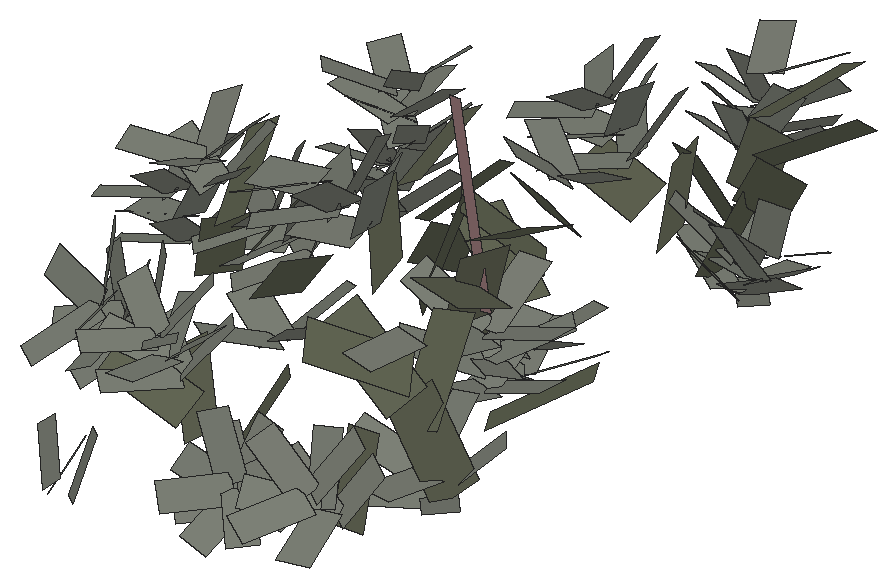
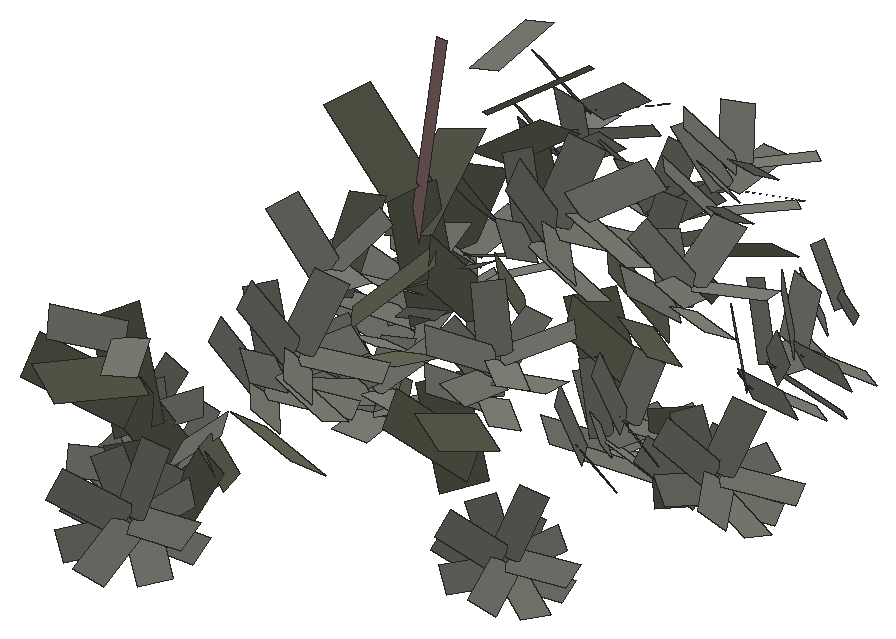
# SketchUp Ruby script. Lengths in inches.
U = 1.inch
M = Sketchup.active_model
def pt(a) = Geom::Point3d.new(a.map { |v| v * U })
def face(e, loops, mat)
  f = e.add_face(loops[0].map { |a| pt(a) })
  loops[1..].each { |l| e.add_face(l.map { |a| pt(a) }).erase! }
  f.material = f.back_material = mat if mat
  f
end
# faces: each face lists its corners as indices into pts; further lists are holes
def faces(e, pts, list, mat = nil) = list.each { |f| face(e, (f[0].is_a?(Array) ? f : [f]).map { |l| l.map { |i| pts[i] } }, mat) }
# xy, xz, yz: faces in a plane at the given z, y or x. An outline is a flat list of corners, or four numbers for a rectangle; further outlines are holes
def ring(l) = l.size == 4 ? [[l[0], l[1]], [l[2], l[1]], [l[2], l[3]], [l[0], l[3]]] : l.each_slice(2).to_a
def flat(e, list, mat, &to3) = list.each { |f| face(e, (f[0].is_a?(Array) ? f : [f]).map { |l| ring(l).map { |u, v| to3.(u, v) } }, mat) }
def xy(e, z, list, mat = nil) = flat(e, list, mat) { |x, y| [x, y, z] }
def xz(e, y, list, mat = nil) = flat(e, list, mat) { |x, z| [x, y, z] }
def yz(e, x, list, mat = nil) = flat(e, list, mat) { |y, z| [x, y, z] }
def lines(e, pts, list) = list.each { |a, b| e.add_line(pt(pts[a]), pt(pts[b])) }
# prism: a flat outline (further loops are holes) pulled along v
def prism(e, loops, v, mat = nil)
  f = face(e, loops, mat); d = Geom::Vector3d.new(v.map { |x| x * U })
  f.pushpull(f.normal.samedirection?(d) ? d.length : -d.length)
end
def box(e, o, s, mat = nil) = prism(e, [[o, [o[0] + s[0], o[1], o[2]], [o[0] + s[0], o[1] + s[1], o[2]], [o[0], o[1] + s[1], o[2]]]], [0, 0, s[2]], mat)
def at(x, y, z, deg = 0) = Geom::Transformation.translation(pt([x, y, z])) * Geom::Transformation.rotation(ORIGIN, Z_AXIS, deg.degrees)
def axes(o, x, y, z) = Geom::Transformation.new([*x, 0, *y, 0, *z, 0, *pt(o).to_a, 1])
def part(name) = M.definitions.add(name)
# library, detail: a bought-in or finely detailed component or shape, given as its bounding box
def library(name, o, s) = part(name).tap { |d| box(d.entities, o, s) }
def detail(e, o, s) = box(e.add_group.entities, o, s)
def put(e, d, t, mat = nil) = e.add_instance(d, t).tap { |i| i.material = mat if mat }
def group(e, t, mat = nil) = e.add_group.tap { |g| g.transformation = t; g.material = mat if mat }.entities
root = M.entities
M.materials.add("tak1dsfasd0f156w").color = [150, 118, 119]
M.materials.add("viburnumblaasdfas0df1w06d").color = [98, 102, 84]
M.materials.add("viburnumbladsadfasdfad0w122").color = [125, 129, 119]
c1 = part("Component\#315")
p = [[0.25,0,0],[2.05,0.01,0.35],[1.81,4.2,1.66],[0,4.19,1.3125]]
faces(c1.entities,p,[[0,1,2,3]],"viburnumbladsadfasdfad0w122")
c2 = part("viburnumblad2")
put(c2.entities,c1,axes([-19.23,-4.49,-32.18],[83.35428,0,0],[0,79.38502,0],[0,0,83.35428]))
c3 = part("Component\#314")
p = [[0.14,0,0],[2.58,0.05,0.25],[2.44,5.11,2.64],[0,5.05,2.39]]
faces(c3.entities,p,[[0,1,2,3]],"viburnumblaasdfas0df1w06d")
c4 = part("viburnumblad1\#2")
put(c4.entities,c3,axes([-37.25,6.23,19.31],[75.98784,0,0],[0,65.50676,0],[0,0,75.98784]))
c5 = part("Component\#337")
p = [[0.6,0,12.07],[1.51,1.22,0.03],[0.91,1.23,0],[0,0,12.04]]
faces(c5.entities,p,[[0,1,2,3]],"tak1dsfasd0f156w")
put(root,c2,axes([1233.48,261.68,34.33],[-0.00995,0.00489,0.00397],[-0.00628,-0.00876,-0.0047],[0.00102,-0.00608,0.00892]))
put(root,c2,axes([1233.86,263.27,33.78],[-0.01153,-0.00217,-0.00126],[0.00257,-0.00998,-0.00587],[-0.00007,-0.00594,0.00905]))
put(root,c2,axes([1227.22,263.09,31.97],[-0.00593,0.00534,0.00783],[-0.0086,-0.00691,-0.00181],[0.00397,-0.00698,0.00778]))
put(root,c2,axes([1232.86,262.36,33.13],[-0.00254,0.00908,0.00688],[-0.01141,-0.00302,-0.00024],[0.00165,-0.00679,0.00837]))
put(root,c2,axes([1227.72,264.1,32.82],[-0.00902,-0.00601,-0.00274],[0.00624,-0.00625,-0.00686],[0.00215,-0.00706,0.0084]))
put(root,c2,axes([1231.99,261.6,34.32],[0.00636,0.00796,0.00575],[-0.00984,0.00398,0.00495],[0.00146,-0.00765,0.00773]))
put(root,c2,axes([1215.61,263.46,29.77],[0.00345,-0.00905,-0.004],[0.00788,-0.00012,0.00668],[-0.00594,-0.00519,0.00581]))
put(root,c2,axes([1227.25,264.68,31.45],[-0.01058,-0.00047,0.0036],[-0.00191,-0.00936,-0.00683],[0.00314,-0.00674,0.00835]))
put(root,c2,axes([1231.93,262.78,35.2],[0.00995,-0.00489,-0.00397],[0.00634,0.00703,0.00672],[-0.00053,-0.00802,0.00751]))
put(root,c2,axes([1214.98,262.74,28.87],[0.00855,0.00051,0.00592],[-0.00403,0.00835,0.00477],[-0.00448,-0.00623,0.00604]))
put(root,c2,axes([1226.24,263.93,31.04],[0.00218,0.00802,0.00747],[-0.00931,-0.0013,0.00412],[0.00416,-0.00766,0.007]))
put(root,c2,axes([1225.95,263.21,32.57],[0.00902,0.00601,0.00274],[-0.00554,0.00435,0.00868],[0.0036,-0.00837,0.00649]))
put(root,c2,axes([1226.29,265,30.18],[-0.0062,0.00558,0.00817],[-0.00774,-0.00622,-0.00163],[0.00397,-0.00698,0.00778]))
put(root,c2,axes([1215.79,263.78,28.39],[0.00848,-0.00604,0.00136],[0.00312,0.00638,0.00815],[-0.00533,-0.00595,0.00568]))
put(root,c2,axes([1231.8,263,33.61],[0.01153,0.00217,0.00126],[-0.00261,0.00855,0.00823],[0.00055,-0.00816,0.00738]))
put(root,c2,axes([1232.29,263.4375,32.28],[0.00611,0.00764,0.00552],[-0.01063,0.0043,0.00535],[0.00146,-0.00765,0.00773]))
put(root,c2,axes([1226.45,264.22,33.43],[0.00593,-0.00534,-0.00783],[0.00931,0.00502,0.00364],[0.00177,-0.00845,0.00711]))
put(root,c2,axes([1226.68,265.32,32.37],[-0.00218,-0.00802,-0.00747],[0.01085,-0.00048,-0.00266],[0.00158,-0.00777,0.00788]))
put(root,c2,axes([1220.38,265.37,37.75],[-0.00773,0.00806,0.00054],[-0.00787,-0.00734,-0.00302],[-0.00183,-0.00247,0.01075]))
put(root,c2,axes([1221.09,266.52,36.78],[-0.01083,0.00076,-0.00267],[-0.00024,-0.01097,-0.00215],[-0.00276,-0.00202,0.01064]))
put(root,c2,axes([1220.6,266.68,38.24],[-0.00759,-0.00699,-0.00431],[0.00733,-0.00841,0.00072],[-0.00369,-0.00233,0.01029]))
put(root,c2,axes([1232.09,264.59,33.1875],[0.01038,-0.0051,-0.00415],[0.00571,0.00633,0.00604],[-0.00053,-0.00802,0.00751]))
put(root,c2,axes([1225.42,264.67,32.17],[0.01058,0.00047,-0.0036],[0.00255,0.00709,0.00842],[0.00261,-0.00869,0.00653]))
put(root,c2,axes([1221.08,266.54,35.28],[-0.00742,0.00774,0.00052],[-0.0085,-0.00793,-0.00326],[-0.00183,-0.00247,0.01075]))
put(root,c2,axes([1225.21,264.99,30.72],[0.0079,0.00633,0.00186],[-0.00554,0.00435,0.00868],[0.00455,-0.00767,0.00675]))
put(root,c2,axes([1220.16,265.82,36.28],[-0.0001,0.01064,0.00343],[-0.01164,0.00037,-0.00146],[-0.00143,-0.00341,0.01055]))
put(root,c4,axes([1231.6875,266,30.82],[0.01273,-0.00184,0.00122],[0.00029,0.0105,0.01027],[-0.0024,-0.00896,0.00784]))
put(root,c2,axes([1220.25,267.68,36.92],[0.0001,-0.01064,-0.00343],[0.01052,-0.00118,0.00394],[-0.00407,-0.00322,0.0099]))
put(root,c2,axes([1219.03,265.7,37.5],[0.00759,0.00699,0.00431],[-0.00801,0.0076,0.00179],[-0.00181,-0.0043,0.01016]))
put(root,c2,axes([1219.25,267,37.98],[0.00773,-0.00806,-0.00054],[0.0072,0.00653,0.00553],[-0.00368,-0.00417,0.0097]))
put(root,c4,axes([1220.77,267.16,32.375],[0.0023,0.0101,0.00657],[-0.0138,0.00343,-0.00044],[-0.0019,-0.0063,0.01035]))
put(root,c2,axes([1219.1875,266.71,36.29],[0.01083,-0.00076,0.00267],[-0.0004,0.00932,0.00428],[-0.00274,-0.00461,0.00981]))
put(root,c2,axes([1233.8,270.26,40.56],[-0.01204,0.00026,0.00058],[-0.00039,-0.0134,-0.00212],[0.00055,-0.00198,0.01239]))
put(root,c2,axes([1219.7,266.74,35.01],[0.00793,0.00729,0.0045],[-0.00721,0.00684,0.00161],[-0.00181,-0.0043,0.01016]))
put(root,c2,axes([1219.8125,267.84,35.5],[0.00743,-0.00696,-0.00145],[0.0072,0.00653,0.00553],[-0.00282,-0.00502,0.00959]))
put(root,c4,axes([1233.05,270.12,37.29],[-0.00623,0.01061,0.0062],[-0.01365,-0.00831,0.0005],[0.00356,-0.0051,0.0123]))
put(root,c4,axes([1220.29,268.43,30.54],[0.01004,0.00303,0.00636],[-0.00636,0.01197,0.00433],[-0.00443,-0.0059,0.0098]))
put(root,c2,axes([1232.98,272.61,31.45],[-0.01249,0.00076,-0.00112],[-0.00058,-0.01239,-0.00197],[-0.00123,-0.0019,0.01236]))
put(root,c4,axes([1221.05,270.45,28.89],[0.00884,-0.00966,0.00214],[0.00883,0.00982,0.0079],[-0.00632,-0.00331,0.01118]))
put(root,c2,axes([1211.15,273.29,34.3],[-0.00449,-0.0055,-0.01006],[0.00843,-0.00922,0.00132],[-0.00807,-0.00651,0.00641]))
put(root,c4,axes([1231.65,270.49,35.17],[0.00552,0.01118,0.00587],[-0.01458,0.00491,0.00435],[0.00124,-0.00686,0.01189]))
put(root,c2,axes([1211.37,272.11,33.3],[-0.00935,0.00836,-0.00053],[-0.00531,-0.00639,-0.00919],[-0.00638,-0.00686,0.0077]))
put(root,c2,axes([1232.68,272.6,29.72],[-0.00853,0.00907,0.00165],[-0.00968,-0.00877,-0.00184],[-0.00017,-0.0024,0.01233]))
put(root,c2,axes([1232.84,273.94,30.15],[-0.00913,-0.008,-0.00324],[0.00831,-0.00942,-0.00017],[-0.00232,-0.00227,0.01214]))
put(root,c2,axes([1212.33,273.7,33.19],[-0.00979,0.00202,-0.00749],[0.00256,-0.01065,-0.00589],[-0.00735,-0.00634,0.0073]))
put(root,c2,axes([1231.66,271.81,31.08],[0.00042,0.01207,0.00346],[-0.01255,0.00034,0.00035],[0.00024,-0.00347,0.01207]))
put(root,c4,axes([1232.73,272.75,29.4],[0.00411,0.01355,0.00465],[-0.01078,-0.00135,0.01345],[0.01091,-0.00609,0.00813]))
put(root,c2,axes([1211.24,274.87,33.31],[0.00344,-0.0098,-0.00674],[0.00895,-0.00296,0.00831],[-0.00812,-0.00729,0.00557]))
put(root,c2,axes([1213.02,274.3125,31.88],[-0.00898,0.00802,-0.00051],[-0.00573,-0.0069,-0.00993],[-0.00638,-0.00686,0.0077]))
put(root,c2,axes([1209.86,273.75,33.51],[0.00935,-0.00836,0.00053],[0.0036,0.00454,0.01078],[-0.00748,-0.0082,0.00525]))
put(root,c2,axes([1211.75,273.18,32.04],[-0.00344,0.0098,0.00674],[-0.01109,0.00113,-0.00697],[-0.00574,-0.00778,0.00739]))
put(root,c2,axes([1210.08,272.57,32.51],[0.00449,0.0055,0.01006],[-0.01013,0.00737,0.00027],[-0.00579,-0.00855,0.00654]))
put(root,c2,axes([1231.21,272.58,29.54],[0.00913,0.008,0.00324],[-0.00792,0.00789,0.00285],[-0.00024,-0.00448,0.01173]))
put(root,c4,axes([1230.63,272.47,33.07],[0.0147,-0.00029,0.00242],[-0.00086,0.01575,0.00709],[-0.00232,-0.00615,0.01338]))
put(root,c2,axes([1231.27,274.27,30.07],[0.00853,-0.00907,-0.00165],[0.009,0.0076,0.00473],[-0.00239,-0.00435,0.01154]))
put(root,c2,axes([1230.79,273.11,31.36],[0.01249,-0.00076,0.00112],[0.00026,0.01157,0.0049],[-0.00133,-0.00485,0.01151]))
put(root,c2,axes([1210.62,274.11,31.875],[0.00979,-0.00202,0.00749],[-0.00391,0.00808,0.00687],[-0.00651,-0.00873,0.00566]))
put(root,c2,axes([1211.43,275.61,31.89],[0.0093,-0.00683,-0.00004],[0.0036,0.00454,0.01078],[-0.00642,-0.00906,0.00528]))
put(root,c2,axes([1211.72,274.65,31.02],[0.00469,0.00575,0.0105],[-0.00912,0.00663,0.00024],[-0.00579,-0.00855,0.00654]))
put(root,c2,axes([1220.53,278.92,41.66],[-0.00996,0.00362,-0.00815],[-0.00316,-0.01285,-0.00186],[-0.00834,0.00054,0.01043]))
put(root,c2,axes([1213.25,279.76,39.86],[-0.01164,-0.00234,-0.00409],[0.00216,-0.01246,0.00098],[-0.00402,0.00034,0.01124]))
put(root,c2,axes([1221.69,280.12,40.53],[-0.00854,-0.00651,-0.00796],[0.00449,-0.01178,0.00482],[-0.00927,0.0004,0.00962]))
put(root,c4,axes([1230.1,281.29,36.25],[-0.0155,-0.00126,0.00308],[0.00163,-0.01831,0.00072],[0.00301,0.00088,0.01554]))
put(root,c2,axes([1221.23,278.5625,39.98],[-0.00554,0.01163,-0.00356],[-0.00953,-0.00658,-0.00667],[-0.00756,-0.00023,0.01102]))
put(root,c2,axes([1213.1875,280.6875,38.52],[-0.00535,-0.00943,-0.00399],[0.00955,-0.00712,0.00396],[-0.00559,-0.00141,0.01047]))
put(root,c2,axes([1212.24,278.58,39.42],[-0.00261,0.01228,0.0004],[-0.01201,-0.00247,-0.00269],[-0.00228,-0.00087,0.01169]))
put(root,c2,axes([1229.85,281.33,34.3],[-0.01323,-0.00019,0.0019],[0.00023,-0.01336,0.00026],[0.00189,0.00029,0.01323]))
put(root,c2,axes([1216.49,280.45,29.84],[-0.01008,0.00703,-0.00261],[-0.00714,-0.01028,-0.00011],[-0.00193,0.00159,0.01172]))
put(root,c2,axes([1222.06,280.88,38.94],[-0.00096,-0.01167,-0.00375],[0.00883,-0.00372,0.00932],[-0.00998,-0.00196,0.00867]))
put(root,c2,axes([1229.51,281.72,31.14],[-0.01229,-0.00021,0.00042],[0.00023,-0.01336,0.00026],[0.00045,0.00027,0.01335]))
put(root,c2,axes([1229.3125,280.67,32.59],[-0.00935,0.00927,0.0023],[-0.00914,-0.00973,0.00201],[0.00303,-0.00016,0.01302]))
put(root,c2,axes([1219.34,278.36,40.59],[0.00212,0.01282,0.00311],[-0.01094,0.00347,-0.00685],[-0.00738,-0.00146,0.01104]))
put(root,c4,axes([1215.92,282.14,31.47],[-0.00759,-0.01277,-0.00082],[0.01374,-0.0085,0.0061],[-0.0047,0.00228,0.01321]))
put(root,c2,axes([1221.78,278.8,38.3],[0.00203,0.01231,0.00299],[-0.01181,0.00375,-0.0074],[-0.00738,-0.00146,0.01104]))
put(root,c2,axes([1211.84,280.76,39.46],[0.00261,-0.01228,-0.0004],[0.01019,0.002,0.00499],[-0.00512,-0.00144,0.01069]))
put(root,c2,axes([1216.47,282.04,29.8125],[-0.00685,-0.0104,-0.00154],[0.00967,-0.00694,0.00401],[-0.00399,0.00118,0.01121]))
put(root,c2,axes([1229.31,282.55,32.74],[-0.00935,-0.00954,0.00039],[0.00874,-0.00859,-0.00062],[0.00075,-0.0002,0.01334]))
put(root,c5,axes([1227.54,280.05,35.54],[1.0472,0,0],[0,1.0472,0],[0,0,1.0472]))
put(root,c2,axes([1220.3125,280.63,39.35],[0.00554,-0.01163,0.00356],[0.00681,0.00581,0.00839],[-0.00964,-0.00181,0.00908]))
put(root,c4,axes([1229.08,282.375,39.14],[-0.00531,-0.01357,0.00158],[0.01582,-0.00598,0.00178],[-0.00086,0.00203,0.01449]))
put(root,c2,axes([1212.16,279.03,37.875],[0.00613,0.00993,0.00305],[-0.0113,0.00738,-0.00131],[-0.00247,-0.00201,0.01151]))
put(root,c4,axes([1227.6875,282.38,32.59],[-0.00382,-0.01538,-0.00062],[0.0121,-0.00355,0.01339],[-0.01131,0.00237,0.01086]))
put(root,c2,axes([1228.49,280.34,34.4],[0,0.0133,0.00135],[-0.0129,-0.00035,0.00349],[0.0035,-0.0013,0.01283]))
put(root,c2,axes([1220.15,279.09,39.07],[0.00854,0.00651,0.00796],[-0.00689,0.01199,-0.00242],[-0.00792,-0.00244,0.01048]))
put(root,c2,axes([1211.9375,280.61,38.01],[0.01052,-0.00734,0.00272],[0.0053,0.00911,0.00408],[-0.00448,-0.00242,0.01081]))
put(root,c2,axes([1211.18,279.48,39.13],[0.01164,0.00234,0.00409],[-0.0032,0.01265,0.00186],[-0.00338,-0.00265,0.01114]))
put(root,c2,axes([1228.89,282.69,34.58],[0,-0.0133,-0.00135],[0.01336,0.00003,-0.00028],[0.00028,-0.00135,0.01329]))
put(root,c2,axes([1221.14,280.34,37.97],[0.01039,-0.00378,0.00851],[0.00094,0.01134,0.00389],[-0.00886,-0.00258,0.00967]))
put(root,c2,axes([1228.62,282.85,31.28],[0,-0.01388,-0.00141],[0.01203,0.00003,-0.00025],[0.00028,-0.00135,0.01329]))
put(root,c2,axes([1214.95,280.42,29.46],[0.00685,0.0104,0.00154],[-0.01034,0.00702,-0.00117],[-0.00153,-0.00054,0.01185]))
put(root,c4,axes([1223.2,279.97,35.24],[0.00849,0.00329,0.01149],[-0.00585,0.01597,-0.00025],[-0.01083,-0.00383,0.0091]))
put(root,c4,axes([1212.54,280.4,34.99],[0.01199,-0.00124,0.00662],[-0.00048,0.01553,0.00369],[-0.00665,-0.00299,0.01093]))
put(root,c4,axes([1213.63,281.83,33.3],[0.0067,-0.01138,0.00383],[0.01125,0.009,0.0069],[-0.00701,-0.00007,0.01111]))
put(root,c2,axes([1227.63,280.9,32.86],[0.00935,0.00954,-0.00039],[-0.00905,0.00903,0.00388],[0.00303,-0.00246,0.01278]))
put(root,c2,axes([1212.76,285.04,34.51],[-0.00608,-0.00542,-0.00802],[0.00543,-0.00975,0.00248],[-0.00802,-0.0025,0.00776]))
put(root,c2,axes([1208.39,284.78,31.62],[-0.00935,-0.0054,-0.00582],[0.00241,-0.00918,0.00416],[-0.00697,0.00288,0.00746]))
put(root,c2,axes([1214.93,282.01,29.43],[0.01008,-0.00703,0.00261],[0.00646,0.01036,0.00294],[-0.0036,-0.00095,0.01134]))
put(root,c4,axes([1224.71,281.56,33.62],[0.00719,-0.00894,0.00913],[0.00526,0.01343,0.009],[-0.01194,-0.00098,0.00844]))
put(root,c2,axes([1213.8,284.91,33.32],[-0.0088,0.00279,-0.00674],[-0.00068,-0.01083,-0.00359],[-0.00727,-0.00236,0.00851]))
put(root,c2,axes([1227.76,282.4,32.97],[0.00935,-0.00927,-0.0023],[0.00999,0.00977,0.00128],[0.00075,-0.00249,0.01311]))
put(root,c2,axes([1207.65,284.54,32.62],[-0.00882,0.00375,-0.00654],[-0.00425,-0.0099,-0.00033],[-0.00607,0.00296,0.00807]))
put(root,c2,axes([1212.6,283.79,33.79],[-0.00637,0.00937,-0.00151],[-0.00692,-0.00583,-0.00699],[-0.0065,-0.00298,0.00892]))
put(root,c2,axes([1206.83,285.4,33.6],[-0.00896,-0.00518,-0.00557],[0.00268,-0.0102,0.00462],[-0.00697,0.00288,0.00746]))
put(root,c4,axes([1209.9,284.91,29.4375],[-0.0079,-0.01009,-0.00146],[0.00852,-0.00752,0.00905],[-0.00687,0.00486,0.00819]))
put(root,c2,axes([1207.8125,283.66,31.45],[-0.00267,0.00936,-0.00422],[-0.0097,-0.00494,-0.00456],[-0.00579,0.00336,0.00814]))
put(root,c2,axes([1227.53,281.7,34.68],[0.01323,0.00019,-0.0019],[0.00023,0.01303,0.00294],[0.00189,-0.00295,0.0129]))
put(root,c2,axes([1227.33,281.74,31.3125],[0.0127,0.00018,-0.00182],[0.00025,0.01408,0.00318],[0.00189,-0.00295,0.0129]))
put(root,c4,axes([1227.47,283.21,28.06],[0.00753,-0.01256,0.00063],[0.01453,0.00876,0.0012],[-0.00121,0,0.01461]))
put(root,c2,axes([1206.16,284.11,33.29],[-0.00351,0.01047,-0.00368],[-0.0097,-0.00494,-0.00456],[-0.00545,0.00224,0.00858]))
put(root,c2,axes([1228.4375,286.24,29.64],[-0.01209,-0.0034,-0.0003],[0.00332,-0.01209,0.00349],[-0.00129,0.00365,0.01095]))
put(root,c2,axes([1228.27,285.6,31.22],[-0.01088,0.00599,-0.0016],[-0.00628,-0.01045,0.00254],[-0.00013,0.00352,0.01104]))
put(root,c2,axes([1207.14,285.72,32.14],[-0.00385,-0.01107,-0.00134],[0.00835,-0.0037,0.00784],[-0.00761,0.00206,0.00711]))
put(root,c2,axes([1214.43,285.03,31.93],[-0.00611,0.009,-0.00145],[-0.00747,-0.0063,-0.00755],[-0.0065,-0.00298,0.00892]))
put(root,c2,axes([1213.11,286.2,33.28],[0.00021,-0.01046,-0.0046],[0.00792,-0.00325,0.00774],[-0.00831,-0.0033,0.00712]))
put(root,c2,axes([1206.36,283.82,31.85],[0.00385,0.01107,0.00134],[-0.00965,0.00395,-0.00558],[-0.00546,0.00115,0.0087]))
put(root,c2,axes([1213.07,284.39,32.39],[-0.00021,0.01046,0.0046],[-0.01011,0.00244,-0.006],[-0.00617,-0.00398,0.00877]))
put(root,c2,axes([1227.81,284.92,29.78],[-0.0033,0.01188,-0.00196],[-0.01112,-0.00285,0.00099],[0.00058,0.00262,0.01122]))
put(root,c2,axes([1228.12,287.16,30.99],[-0.00622,-0.0108,0.00117],[0.01069,-0.00568,0.00296],[-0.00222,0.00293,0.01099]))
put(root,c2,axes([1211.66,285.61,33.77],[0.00637,-0.00937,0.00151],[0.00514,0.00494,0.00894],[-0.00798,-0.0043,0.00697]))
put(root,c2,axes([1207.34,285.37,30.78],[0.00337,-0.01006,0.00353],[0.00874,0.00576,0.00702],[-0.00763,0.00098,0.00722]))
put(root,c2,axes([1211.5,284.37,33.05],[0.00608,0.00542,0.00802],[-0.00721,0.00886,-0.00053],[-0.00646,-0.00478,0.00813]))
put(root,c4,axes([1228.3,286.67,35.03],[-0.00837,0.01093,-0.00027],[-0.01213,-0.00903,0.00454],[0.00324,0.00308,0.01192]))
put(root,c2,axes([1205.82,286.11,32.82],[0.00351,-0.01047,0.00368],[0.00809,0.00534,0.0065],[-0.00763,0.00098,0.00722]))
put(root,c2,axes([1212.28,285.45,32.125],[0.0088,-0.00279,0.00674],[-0.001,0.00912,0.00509],[-0.00721,-0.00491,0.00738]))
put(root,c2,axes([1213.32,286.54,31.8],[0.00662,-0.00815,0.00069],[0.00514,0.00494,0.00894],[-0.00725,-0.00529,0.00709]))
put(root,c4,axes([1228.71,288.53,36.625],[-0.0135,0.00082,0.00242],[0.00046,-0.01443,0.00598],[0.00274,0.00585,0.01119]))
put(root,c2,axes([1206.09,285.25,31.5],[0.00882,-0.00375,0.00654],[0.00302,0.01118,0.0023],[-0.00701,0.00026,0.00774]))
put(root,c2,axes([1205.15,284.8125,32.51],[0.00896,0.00518,0.00557],[-0.00429,0.01059,-0.00268],[-0.00611,0.00033,0.00835]))
put(root,c2,axes([1227.27,287.03,29.47],[0.0033,-0.01188,0.00196],[0.01189,0.00365,0.00167],[-0.00236,0.00179,0.01115]))
put(root,c2,axes([1213.29,285.49,31.15],[0.00634,0.00566,0.00838],[-0.00649,0.00797,-0.00047],[-0.00646,-0.00478,0.00813]))
put(root,c2,axes([1226.69,285.4375,31.14],[0.00622,0.0108,-0.00117],[-0.01091,0.00622,-0.00021],[0.00044,0.00147,0.01138]))
put(root,c4,axes([1226.71,285.72,32.81],[0.00652,0.01335,-0.00071],[-0.01553,0.00758,0.00028],[0.00058,0.00086,0.01356]))
put(root,c2,axes([1226.27,285.77,29.58],[0.01209,0.0034,0.0003],[-0.00342,0.01218,-0.00058],[-0.00049,0.00075,0.01143]))
put(root,c2,axes([1228.375,288.97,39.54],[-0.01136,0.00626,-0.00167],[-0.00561,-0.00886,0.00368],[0.00077,0.00497,0.01057]))
put(root,c2,axes([1226.54,286.99,30.91],[0.01088,-0.00599,0.0016],[0.00606,0.01099,0.00021],[-0.00165,0.00089,0.01133]))
put(root,c2,axes([1228.09,290.45,39.1],[-0.00603,-0.00996,0.00266],[0.01166,-0.00593,0.00316],[-0.00133,0.00444,0.01071]))
put(root,c4,axes([1218.73,290.98,29.85],[-0.00965,-0.00928,0.0022],[0.01068,-0.00958,0.00645],[-0.00246,0.00545,0.01217]))
put(root,c2,axes([1216.57,291.08,38.31],[-0.01113,0.0001,-0.00261],[-0.00085,-0.01106,0.00319],[-0.00248,0.00327,0.01067]))
put(root,c2,axes([1216.61,291.65,36.88],[-0.0072,-0.00751,-0.00155],[0.00713,-0.00775,0.00446],[-0.00433,0.00201,0.01039]))
put(root,c2,axes([1215.66,290.6,39.69],[-0.00749,0.00804,-0.00315],[-0.0085,-0.00761,0.00079],[-0.00154,0.00286,0.01096]))
put(root,c2,axes([1215.96,292,39.52],[-0.00825,-0.0079,-0.00055],[0.00713,-0.00775,0.00446],[-0.00345,0.00288,0.01051]))
put(root,c2,axes([1227.03,288.82,39.67],[0.00561,0.0092,-0.00364],[-0.0108,0.0064,-0.00025],[0.002,0.00408,0.01074]))
put(root,c2,axes([1215.38,290.23,38.18],[0.00053,0.01127,-0.00184],[-0.01136,0.00033,-0.00126],[-0.00119,0.00188,0.01121]))
put(root,c2,axes([1215.52,292.21,37.83],[-0.00053,-0.01127,0.00184],[0.00985,0.00012,0.00361],[-0.0039,0.00191,0.01058]))
put(root,c2,axes([1215.27,290.36,36.66],[0.00792,0.00758,0.00053],[-0.00837,0.00887,-0.00193],[-0.00163,0.00092,0.01128]))
put(root,c2,axes([1215.45,291.8,36.49],[0.00782,-0.00839,0.00329],[0.00709,0.00727,0.00169],[-0.00355,0.00093,0.01083]))
put(root,c4,axes([1216.8,291.6,31.76],[0.00364,-0.01074,0.00535],[0.01254,0.00622,0.00396],[-0.00521,0.00362,0.01082]))
put(root,c2,axes([1214.28,290.86,39.33],[0.00825,0.0079,0.00055],[-0.00775,0.00821,-0.00179],[-0.00163,0.00092,0.01128]))
put(root,c2,axes([1214.59,292.26,39.16],[0.00749,-0.00804,0.00315],[0.00787,0.00807,0.00188],[-0.00355,0.00093,0.01083]))
put(root,c2,axes([1214.62,291.21,37.81],[0.01113,-0.0001,0.00261],[0.00023,0.01199,-0.00051],[-0.00261,0.00052,0.01112]))
put(root,c4,axes([1215.66,290.9375,33.6875],[0.01084,-0.00282,0.00565],[0.00343,0.01413,0.00046],[-0.00557,0.00099,0.01119]))
put(root,c2,axes([1212.72,295.12,29.96],[-0.00996,-0.0034,-0.00378],[0.0004,-0.00774,0.0055],[-0.00482,0.0055,0.00684]))
put(root,c2,axes([1212.1,295.27,30.98],[-0.00747,0.00421,-0.00626],[-0.00602,-0.00754,0.00188],[-0.00396,0.00545,0.00734]))
put(root,c2,axes([1211.94,294.26,30.06],[-0.00059,0.00795,-0.00557],[-0.01005,-0.00269,-0.00267],[-0.00362,0.00574,0.0073]))
put(root,c2,axes([1225.36,296.4375,38.29],[-0.00962,0.00434,-0.00682],[-0.00417,-0.01174,-0.00159],[-0.00692,0.00104,0.01043]))
put(root,c2,axes([1224.49,297.07,39.65],[-0.00913,-0.00526,-0.00683],[0.00354,-0.01136,0.00402],[-0.00787,0.001,0.00974]))
put(root,c2,axes([1211.66,296.39,31.79],[-0.00954,-0.00326,-0.00362],[0.00044,-0.00861,0.00611],[-0.00482,0.0055,0.00684]))
put(root,c2,axes([1211.88,296.33,30.34],[-0.00602,-0.00882,0.00114],[0.00718,-0.00382,0.00749],[-0.0056,0.00489,0.00671]))
put(root,c2,axes([1223.87,295.7,39.15],[-0.00447,0.0114,-0.0028],[-0.00996,-0.00527,-0.00554],[-0.00621,0.00025,0.01092]))
put(root,c2,axes([1210.75,295.38,31.79],[-0.00103,0.00921,-0.00523],[-0.01005,-0.00269,-0.00267],[-0.00353,0.00478,0.00792]))
put(root,c2,axes([1211.85,295.73,29.125],[0.00099,-0.00884,0.00502],[0.00961,0.00407,0.00487],[-0.00586,0.00398,0.00703]))
put(root,c2,axes([1225.83,296.16,36.7],[-0.00429,0.01094,-0.00269],[-0.01076,-0.0057,-0.00599],[-0.00621,0.00025,0.01092]))
put(root,c2,axes([1210.74,294.83,30.49],[0.00602,0.00882,-0.00114],[-0.00807,0.00476,-0.00535],[-0.00378,0.00387,0.00824]))
put(root,c2,axes([1224.97,297.98,38.06],[-0.0033,-0.01178,-0.00285],[0.00874,-0.0044,0.00808],[-0.00849,0.00014,0.00926]))
put(root,c2,axes([1233.92,297.87,32.27],[-0.01012,-0.0002,-0.00445],[-0.00314,-0.00766,0.00749],[-0.00319,0.00804,0.00689]))
put(root,c2,axes([1210.86,297.1,30.98],[0.00103,-0.00921,0.00523],[0.0089,0.00377,0.00451],[-0.00586,0.00398,0.00703]))
put(root,c2,axes([1231.54,298.48,30.07],[-0.01209,0.00339,-0.00041],[-0.00309,-0.0102,0.00689],[0.00151,0.00666,0.01054]))
put(root,c2,axes([1210.79,296.06,29.9],[0.00747,-0.00421,0.00626],[0.0054,0.00929,-0.00022],[-0.00543,0.00331,0.00761]))
put(root,c2,axes([1224.3,295.96,37.47],[0.0033,0.01178,0.00285],[-0.01097,0.00447,-0.0058],[-0.00615,-0.00092,0.01092]))
put(root,c2,axes([1223.36,297.87,38.87],[0.00447,-0.0114,0.0028],[0.00817,0.00518,0.00802],[-0.00843,-0.00103,0.00925]))
put(root,c2,axes([1209.95,296.09,30.99],[0.00954,0.00326,0.00362],[-0.0016,0.00968,-0.00428],[-0.00457,0.00326,0.00811]))
put(root,c2,axes([1232.8,298.21,33.46],[-0.00525,0.00588,-0.00776],[-0.00943,-0.00525,0.0024],[-0.00241,0.00775,0.0075]))
put(root,c4,axes([1226.68,296.35,33.46],[0.00447,0.01094,0.00709],[-0.01215,0.00867,-0.00572],[-0.00776,-0.00379,0.01074]))
put(root,c2,axes([1225.04,298.03,36.375],[0.00493,-0.01032,0.00165],[0.00817,0.00518,0.00802],[-0.0079,-0.00226,0.0095]))
put(root,c2,axes([1232.67,297.21,32.3125],[0.0027,0.00851,-0.00652],[-0.01047,0.00066,-0.00347],[-0.00228,0.00703,0.00822]))
put(root,c2,axes([1231.54,299.91,31.17],[-0.01083,-0.00527,0.00359],[0.00636,-0.00933,0.00551],[0.00035,0.00657,0.01071]))
put(root,c2,axes([1233.35,299.28,32.74],[-0.00906,-0.00616,0.00146],[0.00477,-0.00497,0.00864],[-0.00416,0.00772,0.00674]))
put(root,c2,axes([1232.8,296.6,30.97],[0.0087,0.00591,-0.0014],[-0.00609,0.00723,-0.0073],[-0.00288,0.00629,0.00863]))
put(root,c2,axes([1222.74,296.49,38.36],[0.00913,0.00526,0.00683],[-0.00534,0.01127,-0.00154],[-0.00678,-0.00178,0.01043]))
put(root,c2,axes([1223.7,297.24,37.07],[0.00962,-0.00434,0.00682],[0.00218,0.01069,0.00373],[-0.00772,-0.00183,0.00974]))
put(root,c2,axes([1224.62,296.83,35.9],[0.00954,0.0055,0.00713],[-0.0048,0.01014,-0.00139],[-0.00678,-0.00178,0.01043]))
put(root,c2,axes([1230.88,298.63,31.84],[-0.00627,0.01006,-0.00416],[-0.01061,-0.00457,0.00494],[0.00244,0.00598,0.01078]))
put(root,c2,axes([1230.66,299.89,29.45],[-0.00322,-0.01084,0.00548],[0.01114,-0.00248,0.00163],[-0.00036,0.00575,0.01116]))
put(root,c4,axes([1231.6,300.8,32.78],[-0.01228,-0.00656,0.00533],[0.00976,-0.01204,0.00766],[0.00081,0.00845,0.01225]))
put(root,c2,axes([1230.05,298.01,30.45],[0.00322,0.01084,-0.00548],[-0.01186,0.00402,0.00097],[0.00259,0.00493,0.01126]))
put(root,c2,axes([1232.18,297.91,31.41],[0.01012,0.0002,0.00445],[0.00236,0.00977,-0.0058],[-0.00385,0.00596,0.00848]))
put(root,c4,axes([1229.43,298.97,29.63],[0.00407,-0.01295,0.00616],[0.01043,0.00846,0.01089],[-0.01117,0.00115,0.0098]))
put(root,c4,axes([1227.31,297.49,31.25],[0.00927,0.00064,0.01018],[-0.00266,0.0157,0.00144],[-0.00994,-0.00253,0.00921]))
put(root,c2,axes([1231.6,298.37,32.76],[0.00906,0.00616,-0.00146],[-0.00564,0.00669,-0.00676],[-0.00288,0.00629,0.00863]))
put(root,c2,axes([1230.11,300.57,31],[0.00627,-0.01006,0.00416],[0.01088,0.00589,-0.00218],[-0.0002,0.0047,0.01165]))
put(root,c2,axes([1229.44,299.18,29.92],[0.01209,-0.00339,0.00041],[0.0035,0.01198,-0.00427],[0.00073,0.00402,0.01188]))
put(root,c2,axes([1229.44,299.29,31.67],[0.01083,0.00527,-0.00359],[-0.00609,0.01064,-0.00276],[0.00188,0.00411,0.01172]))
put(root,c4,axes([1227.74,303.33,29.88],[-0.01186,0.00394,-0.00337],[-0.00604,-0.00999,0.00917],[0.00026,0.00862,0.00831]))
put(root,c4,axes([1230.04,302.32,34.92],[0.00185,-0.01141,0.00751],[0.01551,0.00355,0.00158],[-0.0028,0.0071,0.01148]))
put(root,c2,axes([1229.43,303.71,40.12],[0.00655,-0.0105,0.00435],[0.00967,0.00585,-0.00045],[-0.00175,0.00381,0.01184]))
put(root,c2,axes([1228.89,302.29,40.61],[0.01044,0.00574,-0.00186],[-0.00678,0.01138,-0.00292],[0.00034,0.00331,0.01211]))
put(root,c4,axes([1228.97,302.28,37.25],[0.01159,-0.00514,0.00541],[0.00744,0.01388,-0.00276],[-0.00381,0.00452,0.01245]))
put(root,c4,axes([1227.09,305.51,30.42],[-0.01156,-0.00444,0.00366],[0.00659,-0.0076,0.0107],[-0.00137,0.01006,0.00666]))
put(root,c2,axes([1226.38,306.88,32.73],[-0.01201,-0.00131,-0.00224],[-0.00075,-0.00731,0.00743],[-0.00252,0.0083,0.00677]))
put(root,c2,axes([1225.35,306.23,33.1],[0.00059,0.00756,-0.00753],[-0.01174,-0.00037,-0.00119],[-0.00112,0.00828,0.00709]))
put(root,c2,axes([1225.93,307.39,33.87],[-0.00777,0.00552,-0.00673],[-0.00804,-0.00584,0.00423],[-0.00155,0.00808,0.00722]))
put(root,c2,axes([1225.88,308.45,33],[-0.0085,-0.0073,0.00369],[0.00776,-0.00483,0.008],[-0.00353,0.00786,0.00685]))
put(root,c2,axes([1225.49,307.63,31.8125],[-0.0005,-0.0087,0.00708],[0.01199,0.0023,0.00332],[-0.00399,0.00704,0.00741]))
put(root,c2,axes([1225.9,308.82,34.56],[-0.01151,-0.00126,-0.00215],[-0.00083,-0.00812,0.00826],[-0.00252,0.0083,0.00677]))
put(root,c2,axes([1224.67,308.03,34.875],[0.00052,0.00907,-0.00737],[-0.01174,-0.00037,-0.00119],[-0.00118,0.00734,0.00793]))
put(root,c2,axes([1224.3,307.24,33.59],[0.0085,0.0073,-0.00369],[-0.00811,0.00643,-0.0058],[-0.00164,0.00652,0.00849]))
put(root,c2,axes([1224.59,308.41,32.7],[0.00777,-0.00552,0.00673],[0.00812,0.00813,-0.00272],[-0.00362,0.0063,0.00812]))
put(root,c2,axes([1225.11,309.67,33.64],[-0.00052,-0.00907,0.00737],[0.0111,0.00213,0.00308],[-0.00399,0.00704,0.00741]))
put(root,c2,axes([1223.89,308.875,33.96],[0.01151,0.00126,0.00215],[0.0002,0.00988,-0.00637],[-0.00265,0.00609,0.00857]))
